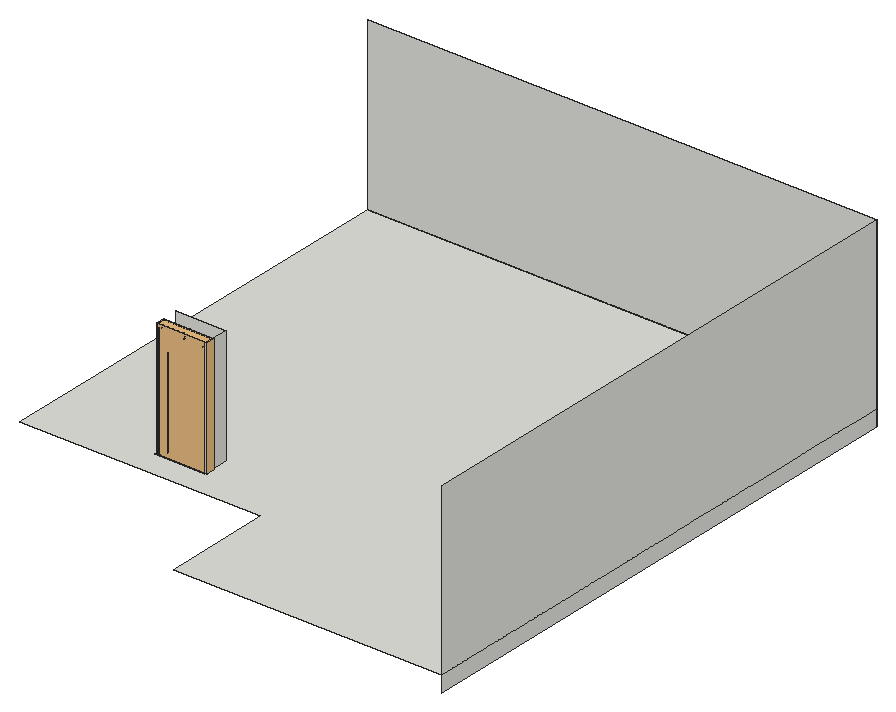
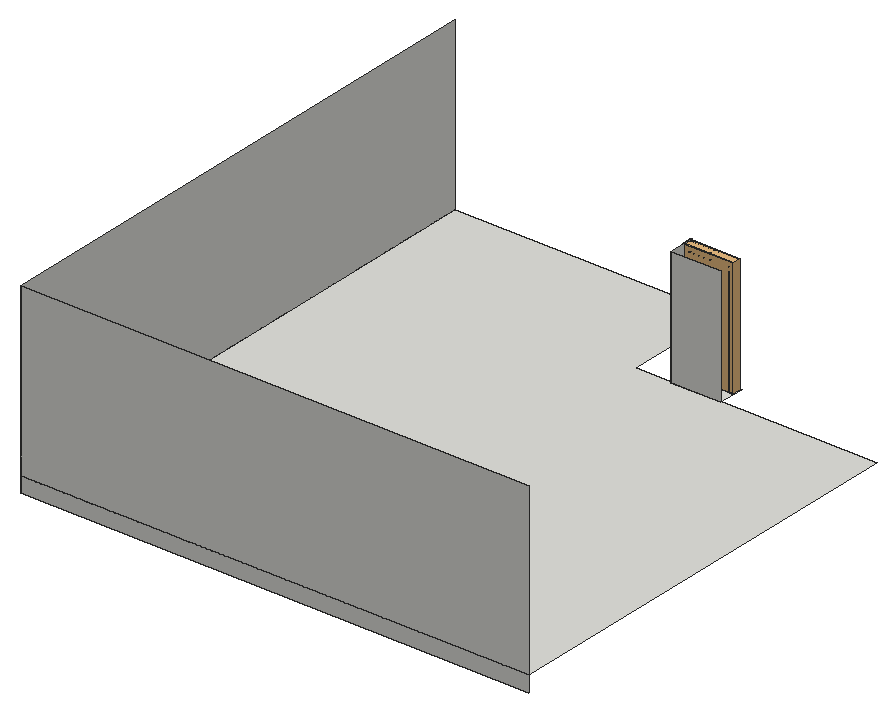
# SketchUp Ruby script. Lengths in inches.
U = 1.inch
M = Sketchup.active_model
def pt(a) = Geom::Point3d.new(a.map { |v| v * U })
def face(e, loops, mat)
  f = e.add_face(loops[0].map { |a| pt(a) })
  loops[1..].each { |l| e.add_face(l.map { |a| pt(a) }).erase! }
  f.material = f.back_material = mat if mat
  f
end
# faces: each face lists its corners as indices into pts; further lists are holes
def faces(e, pts, list, mat = nil) = list.each { |f| face(e, (f[0].is_a?(Array) ? f : [f]).map { |l| l.map { |i| pts[i] } }, mat) }
# xy, xz, yz: faces in a plane at the given z, y or x. An outline is a flat list of corners, or four numbers for a rectangle; further outlines are holes
def ring(l) = l.size == 4 ? [[l[0], l[1]], [l[2], l[1]], [l[2], l[3]], [l[0], l[3]]] : l.each_slice(2).to_a
def flat(e, list, mat, &to3) = list.each { |f| face(e, (f[0].is_a?(Array) ? f : [f]).map { |l| ring(l).map { |u, v| to3.(u, v) } }, mat) }
def xy(e, z, list, mat = nil) = flat(e, list, mat) { |x, y| [x, y, z] }
def xz(e, y, list, mat = nil) = flat(e, list, mat) { |x, z| [x, y, z] }
def yz(e, x, list, mat = nil) = flat(e, list, mat) { |y, z| [x, y, z] }
def lines(e, pts, list) = list.each { |a, b| e.add_line(pt(pts[a]), pt(pts[b])) }
# prism: a flat outline (further loops are holes) pulled along v
def prism(e, loops, v, mat = nil)
  f = face(e, loops, mat); d = Geom::Vector3d.new(v.map { |x| x * U })
  f.pushpull(f.normal.samedirection?(d) ? d.length : -d.length)
end
def box(e, o, s, mat = nil) = prism(e, [[o, [o[0] + s[0], o[1], o[2]], [o[0] + s[0], o[1] + s[1], o[2]], [o[0], o[1] + s[1], o[2]]]], [0, 0, s[2]], mat)
def at(x, y, z, deg = 0) = Geom::Transformation.translation(pt([x, y, z])) * Geom::Transformation.rotation(ORIGIN, Z_AXIS, deg.degrees)
def axes(o, x, y, z) = Geom::Transformation.new([*x, 0, *y, 0, *z, 0, *pt(o).to_a, 1])
def part(name) = M.definitions.add(name)
# library, detail: a bought-in or finely detailed component or shape, given as its bounding box
def library(name, o, s) = part(name).tap { |d| box(d.entities, o, s) }
def detail(e, o, s) = box(e.add_group.entities, o, s)
def put(e, d, t, mat = nil) = e.add_instance(d, t).tap { |i| i.material = mat if mat }
def group(e, t, mat = nil) = e.add_group.tap { |g| g.transformation = t; g.material = mat if mat }.entities
root = M.entities
M.materials.add("Material \#0").color = [86, 53, 35]
M.materials.add("Material \#1").color = [140, 140, 140]
c1 = part("3DGeom~19_Defintion")
xy(c1.entities,0,[[-6.28,-215.79,-994.45,-208.55,-13.52,-208.55],[-994.45,-215.79,-994.45,-208.55,-6.28,-215.79],[-6.28,-215.79,-13.52,-208.55,-13.52,0],[-6.28,-215.79,-13.52,0,-6.28,0],[-13.52,0,-13.52,208.55,-6.28,215.79],
  [-13.52,0,-6.28,215.79,-6.28,0],[-994.45,208.55,-6.28,215.79,-13.52,208.55],[-994.45,208.55,-994.45,215.79,-6.28,215.79]],"Material \#0")
p = [[-13.52,-208.55,0],[-994.45,-208.55,0],[-994.45,-207.81,0.07],[-14.25,-207.81,0.07],[-13.52,-208.55,0],[-14.25,-207.81,0.07],
  [-14.25,0,0.07],[-13.52,0,0],[-13.52,208.55,0],[-14.25,207.81,0.07],[-13.52,208.55,0],[-14.25,207.81,0.07],
  [-994.45,207.81,0.07],[-994.45,208.55,0],[-994.45,-207.21,0.27],[-994.45,-207.21,0.27],[-14.86,-207.21,0.27],[-14.86,-207.21,0.27],
  [-14.86,0,0.27],[-14.86,0,0.27],[-14.86,0,0.27],[-14.86,0,0.27],[-14.86,207.21,0.27],[-14.86,207.21,0.27],
  [-994.45,207.21,0.27],[-994.45,207.21,0.27],[-14.86,-207.21,0.27],[-994.45,-207.21,0.27],[-994.45,-206.74,0.6],[-15.33,-206.74,0.6],
  [-14.86,-207.21,0.27],[-15.33,-206.74,0.6],[-15.33,0,0.6],[-14.86,0,0.27],[-14.86,207.21,0.27],[-15.33,206.74,0.6],
  [-14.86,207.21,0.27],[-15.33,206.74,0.6],[-994.45,206.74,0.6],[-994.45,207.21,0.27],[-994.45,-206.4,1.07],[-15.66,-206.4,1.07],
  [-15.66,-206.4,1.07],[-15.66,0,1.07],[-15.66,206.4,1.07],[-15.66,206.4,1.07],[-994.45,206.4,1.07],[-994.45,-206.2,1.68],
  [-15.86,-206.2,1.68],[-15.86,-206.2,1.68],[-15.86,0,1.68],[-15.86,206.2,1.68],[-15.86,206.2,1.68],[-994.45,206.2,1.68],
  [-994.45,-206.13,2.41],[-15.93,-206.13,2.41],[-15.93,-206.13,2.41],[-15.93,0,2.41],[-15.93,206.13,2.41],[-15.93,206.13,2.41],
  [-994.45,206.13,2.41],[-994.45,-206.13,71.16],[-994.45,-206.22,71.59],[-15.79,-206.28,71.53],[-15.79,-206.28,71.53],[-15.84,0,71.59],
  [-15.93,0,71.16],[-15.79,206.28,71.53],[-15.79,206.28,71.53],[-994.45,206.22,71.59],[-994.45,206.13,71.16],[-15.79,-206.28,71.53],
  [-994.45,-206.48,71.84],[-994.45,-206.9,71.93],[-15.16,-206.9,71.93],[-15.79,-206.28,71.53],[-15.79,-206.28,71.53],[-15.16,-206.9,71.93],
  [-15.16,0,71.93],[-994.45,-206.48,71.84],[-15.59,0,71.84],[-15.79,-206.28,71.53],[-15.59,0,71.84],[-15.79,206.28,71.53],
  [-15.16,206.9,71.93],[-15.59,0,71.84],[-15.79,206.28,71.53],[-994.45,206.48,71.84],[-15.79,206.28,71.53],[-15.16,206.9,71.93],
  [-994.45,206.9,71.93],[-994.45,206.48,71.84],[-15.79,206.28,71.53],[-994.45,-227.27,72.01],[5.41,-227.47,72.33],[4.78,-226.84,71.93],
  [4.78,-226.84,71.93],[5.41,-227.47,72.33],[5.21,0,72.01],[-994.45,-226.84,71.93],[-994.45,-227.27,72.01],[5.21,0,72.01],
  [4.78,0,71.93],[4.78,226.84,71.93],[5.21,0,72.01],[5.21,0,72.01],[5.41,227.47,72.33],[4.78,226.84,71.93],
  [5.41,227.47,72.33],[-994.45,227.27,72.01],[-994.45,227.27,72.01],[-994.45,226.84,71.93],[-994.45,-227.27,72.01],[-994.45,-227.53,72.27],
  [5.41,-227.47,72.33],[5.41,-227.47,72.33],[5.47,0,72.27],[5.21,0,72.01],[5.41,227.47,72.33],[5.41,227.47,72.33],
  [-994.45,227.53,72.27],[-994.45,227.27,72.01],[-994.45,-227.61,72.7],[-994.45,-227.61,74.4375],[-994.45,-227.61,74.4375],[5.55,-227.61,74.4375],
  [5.55,-227.61,74.4375],[5.55,0,74.4375],[5.55,0,72.7],[5.55,227.61,74.4375],[5.55,227.61,74.4375],[-994.45,227.61,74.4375],
  [-994.45,227.61,74.4375],[-994.45,227.61,72.7]]
faces(c1.entities,p,[[0,1,2],[2,3,0],[4,5,6],[6,7,4],[8,7,6],[6,9,8],[10,11,12],[12,13,10],
  [3,2,14],[15,16,3],[5,17,18],[19,6,5],[9,6,20],[21,22,9],[11,23,24],[25,12,11],
  [26,27,28],[28,29,26],[30,31,32],[32,33,30],[34,33,32],[32,35,34],[36,37,38],[38,39,36],
  [29,28,40],[40,41,29],[31,42,43],[43,32,31],[35,32,43],[43,44,35],[37,45,46],[46,38,37],
  [41,40,47],[47,48,41],[42,49,50],[50,43,42],[44,43,50],[50,51,44],[45,52,53],[53,46,45],
  [48,47,54],[54,55,48],[49,56,57],[57,50,49],[51,50,57],[57,58,51],[52,59,60],[60,53,52],
  [61,62,63],[64,65,66],[66,65,67],[68,69,70],[71,72,73],[73,74,75],[76,77,78],[62,79,63],
  [78,80,76],[81,82,65],[83,80,78],[78,84,83],[65,85,86],[68,87,69],[88,89,90],[90,91,92],
  [93,94,95],[96,97,98],[95,99,100],[101,102,96],[103,102,104],[105,106,103],[107,108,109],[110,111,107],
  [112,113,114],[115,116,117],[117,116,118],[119,120,121],[114,122,123],[124,125,114],[113,122,114],[115,126,127],
  [127,128,115],[115,128,116],[118,128,127],[127,129,118],[116,128,118],[119,130,131],[132,133,119],[119,133,120]],"Material \#0")
c2 = part("3DGeom~15_Defintion")
xy(c2.entities,0,[[-961.58,-251.9,-958.5,-248.8125,-961.58,-237.8],[-961.58,-251.9,28.8,-248.8125,-958.5,-248.8125],[-961.58,-251.9,36.25,-251.9,28.8,-248.8125],[36.25,-251.9,19.98,-239.99,28.8,-248.8125],[36.25,-251.9,22.16,-237.8,19.98,-239.99],
  [-958.5,-248.8125,-958.5,-237.8,-961.58,-237.8],[19.98,-239.99,22.16,-237.8,3.36,-223.37],[-958.5,-237.8,-958.5,-223.37,-961.58,-220.28],[-961.58,-237.8,-958.5,-237.8,-961.58,-220.28],[22.16,-237.8,4.64,-220.28,3.36,-223.37],
  [-958.5,-223.37,4.64,-220.28,-961.58,-220.28],[-958.5,-223.37,3.36,-223.37,4.64,-220.28],[5.29,-219.63,8.375,-218.35,5.29,0],[8.375,-218.35,8.375,0,5.29,0],[5.29,0,8.375,0,5.29,219.63],
  [8.375,0,8.375,218.35,5.29,219.63],[8.375,218.35,22.8125,237.15,5.29,219.63],[-961.58,220.28,-958.5,223.37,-961.58,237.8],[-961.58,220.28,3.36,223.37,-958.5,223.37],[-961.58,220.28,4.64,220.28,3.36,223.37],
  [4.64,220.28,19.98,239.99,3.36,223.37],[4.64,220.28,22.16,237.8,19.98,239.99],[-958.5,223.37,-958.5,237.8,-961.58,237.8],[-958.5,237.8,-958.5,248.8125,-961.58,251.9],[-961.58,237.8,-958.5,237.8,-961.58,251.9],
  [22.16,237.8,28.8,248.8125,19.98,239.99],[22.16,237.8,36.25,251.9,28.8,248.8125],[-958.5,248.8125,36.25,251.9,-961.58,251.9],[-958.5,248.8125,28.8,248.8125,36.25,251.9]],"Material \#0")
xy(c2.entities,7.48,[[-962.79,-238.36,23.37,-238.36,-962.79,-219.67],[23.37,-238.36,4.67,-219.67,-962.79,-219.67],[23.37,-238.36,23.37,0,4.67,-219.67],[4.67,-219.67,23.37,0,4.67,0],[23.37,0,23.37,238.36,4.67,219.67],
  [4.67,0,23.37,0,4.67,219.67],[-962.79,219.67,23.37,238.36,-962.79,238.36],[-962.79,219.67,4.67,219.67,23.37,238.36]],"Material \#0")
xy(c2.entities,63.5625,[[-962.79,-238.36,-962.79,-219.67,4.67,-219.67],[-962.79,-238.36,4.67,-219.67,23.37,-238.36],[23.37,-238.36,4.67,-219.67,23.37,0],[4.67,-219.67,4.67,0,23.37,0],[23.37,0,4.67,219.67,23.37,238.36],
  [4.67,0,4.67,219.67,23.37,0],[-962.79,219.67,-962.79,238.36,4.67,219.67],[4.67,219.67,-962.79,238.36,23.37,238.36]],"Material \#0")
xy(c2.entities,69.64,[[-962.79,-219.62,4.63,-219.62,-962.79,-200.32],[4.63,-219.62,-14.68,-200.32,-962.79,-200.32],[4.63,-219.62,4.63,0,-14.68,-200.32],[-14.68,-200.32,4.63,0,-14.68,0],[-14.68,0,4.63,0,-14.68,200.32],
  [4.63,0,4.63,219.62,-14.68,200.32],[-962.79,200.32,-14.68,200.32,4.63,219.62],[-962.79,200.32,4.63,219.62,-962.79,219.62]],"Material \#0")
xy(c2.entities,71.04,[[-961.58,-251.9,-958.5,-248.8125,28.8,-248.8125],[-961.58,-251.9,-961.58,-237.8,-958.5,-248.8125],[-961.58,-251.9,28.8,-248.8125,36.25,-251.9],[36.25,-251.9,19.98,-239.99,22.16,-237.8],[36.25,-251.9,28.8,-248.8125,19.98,-239.99],
  [-958.5,-248.8125,-961.58,-237.8,-958.5,-237.8],[19.98,-239.99,3.36,-223.37,22.16,-237.8],[-958.5,-237.8,-961.58,-220.28,-958.5,-223.37],[-961.58,-237.8,-961.58,-220.28,-958.5,-237.8],[22.16,-237.8,3.36,-223.37,4.64,-220.28],
  [-958.5,-223.37,-961.58,-220.28,4.64,-220.28],[-958.5,-223.37,4.64,-220.28,3.36,-223.37],[5.29,-219.63,5.29,0,8.375,-218.35],[8.375,-218.35,5.29,0,8.375,0],[5.29,0,5.29,219.63,8.375,0],
  [8.375,0,5.29,219.63,8.375,218.35],[8.375,218.35,5.29,219.63,22.8125,237.15],[-961.58,220.28,-958.5,223.37,3.36,223.37],[-961.58,220.28,-961.58,237.8,-958.5,223.37],[-961.58,220.28,3.36,223.37,4.64,220.28],
  [4.64,220.28,3.36,223.37,19.98,239.99],[4.64,220.28,19.98,239.99,22.16,237.8],[-958.5,223.37,-961.58,237.8,-958.5,237.8],[-958.5,237.8,-961.58,251.9,-958.5,248.8125],[-961.58,237.8,-961.58,251.9,-958.5,237.8],
  [22.16,237.8,19.98,239.99,28.8,248.8125],[22.16,237.8,28.8,248.8125,36.25,251.9],[-958.5,248.8125,-961.58,251.9,36.25,251.9],[-958.5,248.8125,36.25,251.9,28.8,248.8125]],"Material \#0")
xz(c2.entities,-238.36,[[-962.79,63.5625,23.37,63.5625,23.37,72.07],[-962.79,63.5625,23.37,72.07,-962.79,72.07]],"Material \#0")
xz(c2.entities,-219.67,[[-962.79,7.48,4.67,7.48,-962.79,63.5625],[4.67,7.48,4.67,63.5625,-962.79,63.5625]],"Material \#0")
xz(c2.entities,219.67,[[-962.79,7.48,-962.79,63.5625,4.67,7.48],[4.67,7.48,-962.79,63.5625,4.67,63.5625]],"Material \#0")
xz(c2.entities,238.36,[[-962.79,63.5625,-962.79,72.07,23.37,72.07],[-962.79,63.5625,23.37,72.07,23.37,63.5625]],"Material \#0")
yz(c2.entities,4.67,[[-219.67,7.48,0,7.48,-219.67,63.5625],[0,7.48,0,63.5625,-219.67,63.5625],[0,7.48,219.67,63.5625,0,63.5625],[0,7.48,219.67,7.48,219.67,63.5625]],"Material \#0")
yz(c2.entities,23.37,[[-238.36,63.5625,0,63.5625,-238.36,72.07],[0,63.5625,0,72.07,-238.36,72.07],[0,63.5625,238.36,63.5625,238.36,72.07],[0,63.5625,238.36,72.07,0,72.07]],"Material \#0")
p = [[36.9,-251.24,0],[37.21,0,-0.16],[34.125,0,-0.14],[36.9,251.24,0],[33.83,243.81,0.02],[33.83,-243.8,0.02],
  [22.8125,-237.15,0],[24.99,-234.97,-0.01],[5.375,-220.37,0],[23.37,-238.36,7.48],[4.67,-219.67,7.48],[4.67,-219.67,7.48],
  [23.37,-238.36,7.48],[23.37,-238.36,0],[4.67,-219.67,7.48],[23.37,-238.36,0],[5.375,-220.37,0],[5.375,-220.37,0],
  [23.37,-238.36,0],[5.29,-219.63,0],[8.375,-218.35,0],[-15.36,-199.64,1.62],[4.67,-219.67,7.48],[5.375,-220.37,0],
  [-13.8,-201.19,0.06],[5.375,-220.37,0],[5.375,-220.37,0],[-14.84,-200.15,0.58],[5.375,-220.37,0],[-13.8,-201.19,0.06],
  [-6.08,-208.92,0],[5.375,-220.37,0],[-13.8,-201.19,0.06],[-6.08,-208.92,0],[-13.8,-201.19,0.06],[5.375,-220.37,0],
  [-6.08,-208.92,0],[-13.8,-201.19,0.06],[-13.09,-201.91,0],[-6.08,-208.92,0],[-13.09,-201.91,0],[-13.8,-201.19,0.06],
  [-15.36,199.64,1.62],[4.67,219.67,7.48],[5.375,220.37,0],[-13.8,201.19,0.06],[5.375,220.37,0],[5.375,220.37,0],
  [4.67,219.67,7.48],[-14.84,200.15,0.58],[5.375,220.37,0],[-13.8,201.19,0.06],[-6.08,208.92,0],[-13.09,201.91,0],
  [-13.8,201.19,0.06],[-6.08,208.92,0],[-13.8,201.19,0.06],[5.375,220.37,0],[-6.08,208.92,0],[5.375,220.37,0],
  [-13.8,201.19,0.06],[-6.08,208.92,0],[-13.8,201.19,0.06],[-13.09,201.91,0],[8.375,218.35,0],[24.99,234.97,-0.01],
  [22.8125,237.15,0],[23.37,238.36,7.48],[23.37,238.36,0],[23.37,238.36,0],[5.375,220.37,0],[5.375,220.37,0],
  [23.37,238.36,7.48],[4.67,219.67,7.48],[5.375,220.37,0],[23.37,238.36,0],[23.37,238.36,7.48],[-13.8,-201.19,0.06],
  [-14.84,-200.15,0.58],[-14.38,-200.61,0.26],[-13.8,-201.19,0.06],[-13.8,-201.19,0.06],[-14.38,-200.61,0.26],[-13.8,201.19,0.06],
  [-14.84,200.15,0.58],[-13.8,201.19,0.06],[-14.38,200.61,0.26],[-14.38,200.61,0.26],[-13.8,201.19,0.06],[4.63,-219.62,69.64],
  [4.63,-219.62,69.64],[-15.42,-199.57,9.43],[-15.36,-199.64,1.62],[-15.16,-199.83,1.04],[-15.16,-199.83,1.04],[-15.16,199.83,1.04],
  [-15.36,199.64,1.62],[-15.16,199.83,1.04],[-15.42,199.57,9.43],[4.63,219.62,69.64],[4.67,219.67,7.48],[4.63,219.62,69.64],
  [4.63,-219.62,69.64],[4.67,-219.67,63.5625],[4.67,-219.67,63.5625],[4.67,-219.67,7.48],[-15.28,-199.71,69.25],[4.63,-219.62,69.64],
  [-15.42,-199.57,9.43],[-15.28,-199.71,69.25],[-15.42,-199.57,2.34],[-15.42,-199.57,2.34],[-15.42,199.57,2.34],[-15.42,199.57,9.43],
  [-15.28,199.71,69.25],[-15.28,199.71,69.25],[4.63,219.62,69.64],[4.63,219.62,69.64],[4.67,219.67,63.5625],[4.67,219.67,63.5625],
  [-15.42,199.57,2.34],[4.67,-219.67,63.5625],[4.63,-219.62,69.64],[4.67,219.67,7.48],[4.67,219.67,63.5625],[4.63,219.62,69.64],
  [4.63,-219.62,69.64],[-15.28,-199.71,69.25],[-15.28,-199.71,69.25],[-15.42,-199.57,48.99],[-15.42,-199.57,48.99],[-15.28,-199.71,69.25],
  [-15.42,199.57,48.99],[-15.28,199.71,69.25],[-15.28,199.71,69.25],[-15.42,199.57,48.99],[4.63,219.62,69.64],[4.63,-219.62,69.64],
  [23.37,-238.36,72.07],[4.67,-219.67,63.5625],[4.67,-219.67,63.5625],[23.37,-238.36,63.5625],[23.37,-238.36,72.07],[4.67,-219.67,63.5625],
  [5.24,-220.23,70.03],[23.37,-238.36,72.07],[23.37,-238.36,63.5625],[4.67,-219.67,63.5625],[4.67,-219.67,63.5625],[4.63,-219.62,69.64],
  [4.63,219.62,69.64],[23.37,238.36,72.07],[4.67,219.67,63.5625],[4.67,219.67,63.5625],[5.24,220.23,70.03],[4.63,219.62,69.64],
  [23.37,238.36,63.5625],[4.67,219.67,63.5625],[4.67,219.67,63.5625],[23.37,238.36,63.5625],[23.37,238.36,72.07],[4.67,219.67,63.5625],
  [23.37,238.36,72.07],[4.63,-219.62,69.64],[-14.68,-200.32,69.64],[-15.28,-199.71,69.25],[-15.28,-199.71,69.25],[-14.68,-200.32,69.64],
  [4.63,-219.62,69.64],[-15.28,199.71,69.25],[-14.68,200.32,69.64],[4.63,219.62,69.64],[4.63,219.62,69.64],[-14.68,200.32,69.64],
  [4.63,-219.62,69.64],[5.24,-220.23,70.03],[23.37,-238.36,72.07],[4.63,219.62,69.64],[5.24,220.23,70.03],[5.375,-220.37,72.07],
  [5.375,-220.37,72.07],[23.37,-238.36,72.07],[5.375,220.37,72.07],[23.37,238.36,72.07],[5.375,220.37,72.07],[33.83,-243.8,71.03],
  [36.9,-251.24,71.04],[22.8125,-237.15,71.04],[34.125,0,71.19],[37.21,0,71.2],[24.99,-234.97,71.05],[5.29,-219.63,71.04],
  [8.375,-218.35,71.04],[33.83,243.81,71.03],[36.9,251.24,71.04],[22.8125,237.15,71.04],[24.99,234.97,71.05],[8.375,218.35,71.04]]
faces(c2.entities,p,[[0,1,2],[1,3,4],[4,2,1],[2,5,0],[6,0,5],[5,7,6],[8,9,10],[11,12,13],
  [14,15,16],[17,18,9],[19,6,7],[7,20,19],[21,22,23],[24,21,25],[26,10,27],[28,27,29],
  [30,31,32],[33,34,35],[36,37,38],[39,40,41],[42,43,44],[45,42,46],[47,48,49],[50,49,51],
  [52,53,54],[55,56,57],[58,59,60],[61,62,63],[64,65,66],[43,67,68],[43,69,70],[71,72,73],
  [74,75,76],[3,66,65],[65,4,3],[77,78,21],[27,79,80],[81,82,78],[83,84,42],[85,86,84],
  [49,87,88],[10,89,27],[90,91,27],[92,93,27],[91,92,27],[78,94,21],[84,95,42],[96,97,49],
  [98,96,49],[99,98,49],[100,101,49],[21,102,103],[21,104,105],[21,106,107],[21,108,109],[91,110,92],
  [21,111,108],[42,112,113],[42,113,114],[42,115,116],[42,117,118],[42,119,43],[98,120,96],[10,121,122],
  [123,124,125],[126,127,91],[128,129,91],[108,130,131],[113,132,133],[134,135,98],[136,134,98],[137,138,139],
  [140,141,142],[143,142,144],[145,146,147],[148,144,149],[150,151,152],[153,154,155],[151,156,157],[158,159,160],
  [161,162,154],[163,164,165],[166,167,168],[169,170,171],[172,173,134],[174,175,176],[177,178,151],[142,179,144],
  [175,180,181],[178,182,151],[183,184,154],[185,186,187],[186,185,188],[188,189,186],[187,190,185],[190,187,191],
  [191,192,190],[189,188,193],[193,194,189],[195,196,197],[196,195,194],[194,193,196]],"Material \#0")
c3 = part("3DGeom~22_Defintion")
xz(c3.entities,-210.625,[[-1016.13,2.47,-1016.13,9.96,-16.28,2.47],[-16.28,2.47,-1016.13,9.96,-16.28,9.96],[-1016.13,9.96,-1016.13,51.7,-16.28,51.7],[-1016.13,9.96,-16.28,51.7,-16.28,9.96],[-1016.13,51.7,-1016.13,72.71,-16.28,51.7]],"Material \#0")
xz(c3.entities,210.625,[[-1016.13,2.47,-16.28,2.47,-1016.13,9.96],[-16.28,2.47,-16.28,9.96,-1016.13,9.96],[-1016.13,9.96,-16.28,51.7,-1016.13,51.7],[-1016.13,9.96,-16.28,9.96,-16.28,51.7],[-1016.13,51.7,-16.28,51.7,-1016.13,72.71]],"Material \#0")
yz(c3.entities,-16.28,[[-210.625,2.47,-210.625,9.96,0,9.96],[-210.625,2.47,0,9.96,0,2.47],[0,2.47,0,9.96,210.625,2.47],[210.625,2.47,0,9.96,210.625,9.96],[-210.625,9.96,-210.625,51.7,0,51.7],
  [-210.625,9.96,0,51.7,0,9.96],[0,9.96,0,51.7,210.625,9.96],[210.625,9.96,0,51.7,210.625,51.7],[-210.625,51.7,0,72.71,0,51.7],[0,51.7,0,72.71,210.625,51.7]],"Material \#0")
p = [[-1016.13,-210.625,72.71],[-16.13,-210.77,73.09],[-16.28,-210.625,51.7],[-16.28,-210.625,51.7],[-16.13,-210.77,73.09],[-16.28,0,72.71],
  [-16.13,210.77,73.09],[-16.28,210.625,51.7],[-16.28,210.625,51.7],[-16.13,210.77,73.09],[-1016.13,210.625,72.71]]
faces(c3.entities,p,[[0,1,2],[3,4,5],[5,6,7],[8,9,10]],"Material \#0")
c4 = library("3DGeom~16_Defintion",[-962.62,-252.34,-11.22],[1000,504.68,93.46])
c5 = part("3DGeom~17_Defintion")
yz(c5.entities,-1908.8,[[-436.03,-21.87,-436.73,-21.5,-435.91,-21.83],[436.03,-21.87,435.91,-21.83,436.73,-21.5],[-435.91,-21.83,-436.73,-21.5,-436.15,-21.125],[-435.91,-21.83,-436.15,-21.125,-435.87,-21.72],[435.91,-21.83,435.87,-21.72,436.15,-21.125],
  [435.91,-21.83,436.15,-21.125,436.73,-21.5],[-436.73,-21.5,-484.73,-21.37,-436.15,-1.11],[-471.46,-21.5,-484.73,-21.37,-436.73,-21.5],[-477.2,-21.5,-484.73,-21.37,-471.46,-21.5],[-481.82,-21.5,-484.73,-21.37,-477.2,-21.5],
  [-436.73,-21.5,-436.15,-1.11,-436.15,-21.125],[436.73,-21.5,436.15,-21.125,471.46,-21.5],[471.46,-21.5,436.15,-21.125,477.2,-21.5],[477.2,-21.5,436.15,-21.125,499.98,-0.85],[477.2,-21.5,499.98,-0.85,481.82,-21.5],
  [481.82,-21.5,487.35,-21,484.73,-21.37],[481.82,-21.5,491.8,-19.52,487.35,-21],[481.82,-21.5,497.64,-13.67,491.8,-19.52],[481.82,-21.5,499.98,-0.85,497.64,-13.67],[-484.73,-21.37,-498.5,-11.58,-499.84,-0.37],
  [-484.73,-21.37,-499.84,-0.37,-499.4,-0.5],[-484.73,-21.37,-499.4,-0.5,-436.15,-1.11],[-484.73,-21.37,-493.63,-18.42,-498.5,-11.58],[-484.73,-21.37,-489.71,-20.375,-493.63,-18.42],[-484.73,-21.37,-487.35,-21,-489.71,-20.375],
  [436.15,-21.125,436.15,-1.11,436.73,-0.74],[436.15,-21.125,436.73,-0.74,499.98,-0.85],[487.35,-21,491.8,-19.52,489.71,-20.375],[-489.71,-20.375,-491.8,-19.52,-493.63,-18.42],[491.8,-19.52,495.21,-17.08,493.63,-18.42],
  [491.8,-19.52,497.64,-13.67,495.21,-17.08],[-493.63,-18.42,-496.54,-15.5,-498.5,-11.58],[-493.63,-18.42,-495.21,-17.08,-496.54,-15.5],[495.21,-17.08,497.64,-13.67,496.54,-15.5],[-496.54,-15.5,-497.64,-13.67,-498.5,-11.58],
  [497.64,-13.67,499.125,-9.22,498.5,-11.58],[497.64,-13.67,499.625,-3.69,499.125,-9.22],[497.64,-13.67,499.98,-0.85,499.625,-3.69],[-498.5,-11.58,-499.625,-3.69,-499.84,-0.37],[-498.5,-11.58,-499.5,-6.6,-499.625,-3.69],
  [-498.5,-11.58,-499.125,-9.22,-499.5,-6.6],[499.125,-9.22,499.625,-3.69,499.5,-6.6],[-499.625,-3.69,-499.98,-0.85,-500,-0.52],[-499.625,-3.69,-500,-0.52,-499.84,-0.37],[-436.15,-1.11,-499.4,-0.5,-471.46,-0.74],
  [-436.15,-1.11,-471.46,-0.74,-436.73,-0.74],[-436.15,-1.11,-436.73,-0.74,-435.91,-0.41],[-436.15,-1.11,-435.91,-0.41,-435.87,-0.52],[436.15,-1.11,435.87,-0.52,435.91,-0.41],[436.15,-1.11,435.91,-0.41,436.73,-0.74],
  [499.98,-0.85,436.73,-0.74,471.46,-0.74],[499.98,-0.85,471.46,-0.74,499.4,-0.5],[499.98,-0.85,499.4,-0.5,499.96,-0.41],[499.98,-0.85,499.96,-0.41,500,-0.52],[-436.73,-0.74,-436.03,-0.37,-435.91,-0.41],
  [436.73,-0.74,435.91,-0.41,436.03,-0.37],[-500,-0.52,-499.96,-0.41,-499.84,-0.37],[499.4,-0.5,499.84,-0.37,499.96,-0.41],[-499.84,141.21,-499.96,141.25,-499.4,141.35],[-436.03,141.21,-436.73,141.59,-435.91,141.25],
  [436.03,141.21,435.91,141.25,436.73,141.59],[499.84,141.21,484.73,162.21,498.5,152.42],[499.84,141.21,499.4,141.35,484.73,162.21],[499.84,141.21,498.5,152.42,499.625,144.53],[499.84,141.21,499.625,144.53,500,141.37],
  [499.84,141.21,500,141.37,499.96,141.25],[-499.96,141.25,-500,141.37,-499.98,141.69],[-499.96,141.25,-499.98,141.69,-499.4,141.35],[-435.91,141.25,-436.73,141.59,-436.15,141.96],[-435.91,141.25,-436.15,141.96,-435.87,141.37],
  [435.91,141.25,435.87,141.37,436.15,141.96],[435.91,141.25,436.15,141.96,436.73,141.59],[-499.4,141.35,-499.98,141.69,-471.46,141.59],[499.4,141.35,436.15,141.96,484.73,162.21],[499.4,141.35,471.46,141.59,436.15,141.96],
  [500,141.37,499.625,144.53,499.98,141.69],[-436.73,141.59,-499.98,141.69,-436.15,161.97],[-471.46,141.59,-499.98,141.69,-436.73,141.59],[-436.73,141.59,-436.15,161.97,-436.15,141.96],[436.73,141.59,436.15,141.96,471.46,141.59],
  [-499.98,141.69,-477.2,162.34,-436.15,161.97],[-499.98,141.69,-481.82,162.34,-477.2,162.34],[-499.98,141.69,-497.64,154.51,-481.82,162.34],[-499.98,141.69,-499.625,144.53,-497.64,154.51],[436.15,141.96,436.15,161.97,436.73,162.34],
  [436.15,141.96,436.73,162.34,484.73,162.21],[-499.625,144.53,-499.125,150.07,-497.64,154.51],[-499.625,144.53,-499.5,147.44,-499.125,150.07],[499.625,144.53,498.5,152.42,499.5,147.44],[499.5,147.44,498.5,152.42,499.125,150.07],
  [-499.125,150.07,-498.5,152.42,-497.64,154.51],[498.5,152.42,484.73,162.21,493.63,159.26],[498.5,152.42,493.63,159.26,496.54,156.34],[498.5,152.42,496.54,156.34,497.64,154.51],[-497.64,154.51,-491.8,160.36,-481.82,162.34],
  [-497.64,154.51,-495.21,157.92,-491.8,160.36],[-497.64,154.51,-496.54,156.34,-495.21,157.92],[496.54,156.34,493.63,159.26,495.21,157.92],[-495.21,157.92,-493.63,159.26,-491.8,160.36],[493.63,159.26,484.73,162.21,489.71,161.22],
  [493.63,159.26,489.71,161.22,491.8,160.36],[-491.8,160.36,-487.35,161.84,-481.82,162.34],[-491.8,160.36,-489.71,161.22,-487.35,161.84],[489.71,161.22,484.73,162.21,487.35,161.84],[-487.35,161.84,-484.73,162.21,-481.82,162.34],
  [-436.15,161.97,-477.2,162.34,-471.46,162.34],[-436.15,161.97,-471.46,162.34,-436.73,162.34],[-436.15,161.97,-436.73,162.34,-435.91,162.68],[-436.15,161.97,-435.91,162.68,-435.87,162.56],[436.15,161.97,435.87,162.56,435.91,162.68],
  [436.15,161.97,435.91,162.68,436.73,162.34],[484.73,162.21,436.73,162.34,471.46,162.34],[484.73,162.21,471.46,162.34,477.2,162.34],[484.73,162.21,477.2,162.34,481.82,162.34],[-436.73,162.34,-436.03,162.72,-435.91,162.68],
  [436.73,162.34,435.91,162.68,436.03,162.72]],"Material \#0")
c6 = part("3DGeom~18_Defintion")
xz(c6.entities,-241.71,[[-976.3,0,23.7,0,23.7,7.58],[-976.3,0,23.7,7.58,-976.3,7.58]],"Material \#0")
xz(c6.entities,241.71,[[-976.3,0,-976.3,7.58,23.7,7.58],[-976.3,0,23.7,7.58,23.7,0]],"Material \#0")
yz(c6.entities,23.7,[[-241.71,0,0,0,-241.71,7.58],[0,0,0,7.58,-241.71,7.58],[0,0,241.71,0,241.71,7.58],[0,0,241.71,7.58,0,7.58]],"Material \#0")
c7 = part("3DGeom~20_Defintion")
xy(c7.entities,0,[[-976.3,-241.71,-976.3,-223.46,23.7,-241.71],[23.7,-241.71,-976.3,-223.46,5.45,-223.46],[23.7,-241.71,5.45,-223.46,5.45,0],[23.7,-241.71,5.45,0,23.7,0],[-976.3,-223.46,-976.3,-211.85,5.45,-223.46],
  [5.45,-223.46,-976.3,-211.85,-6.16,-211.85],[5.45,-223.46,-6.16,-211.85,-6.16,0],[5.45,-223.46,-6.16,0,5.45,0],[-6.16,0,-6.16,211.85,5.45,223.46],[-6.16,0,5.45,223.46,5.45,0],
  [5.45,0,23.7,241.71,23.7,0],[5.45,0,5.45,223.46,23.7,241.71],[-976.3,211.85,-976.3,223.46,5.45,223.46],[-976.3,211.85,5.45,223.46,-6.16,211.85],[-976.3,223.46,-976.3,241.71,23.7,241.71],
  [-976.3,223.46,23.7,241.71,5.45,223.46]],"Material \#0")
xy(root,0,[[169.98,37.59,360,37.59,360,421.59,0,421.59,0,114.72,169.98,114.72]])
xy(root,12.9,[[95,114.72,130.44,133.09]])
xz(root,117.63,[[101.39,47.08,101.49,47.1,101.39,47.09],[101.39,47.08,101.5,47.09,101.49,47.1],[101.5,47.09,101.59,47.13,101.49,47.1],[101.59,47.12,101.68,47.17,101.68,47.18],[101.68,47.17,101.76,47.24,101.68,47.18],
  [101.43,47.26,101.46,47.27,101.46,47.28],[101.43,47.26,101.46,47.28,101.43,47.27],[101.46,47.27,101.48,47.3,101.46,47.28],[101.46,47.27,101.49,47.29,101.48,47.3],[101.49,47.29,101.51,47.32,101.48,47.3],
  [101.49,47.29,101.52,47.31,101.51,47.32],[101.52,47.31,101.53,47.34,101.51,47.32],[101.52,47.31,101.54,47.34,101.53,47.34],[101.53,47.34,101.54,47.34,101.55,47.375],[101.54,47.34,101.56,47.37,101.55,47.375],
  [101.55,47.59,101.56,47.6,101.53,47.62],[101.56,47.6,101.54,47.625,101.53,47.62],[101.53,47.62,101.54,47.625,101.51,47.64],[101.54,47.625,101.52,47.65,101.51,47.64],[101.51,47.64,101.52,47.65,101.48,47.67],
  [101.52,47.65,101.49,47.68,101.48,47.67],[101.48,47.67,101.49,47.68,101.46,47.68],[101.46,47.68,101.46,47.69,101.43,47.69],[101.46,47.68,101.49,47.68,101.46,47.69],[101.43,47.69,101.46,47.69,101.43,47.7]],"Material \#1")
xz(root,133.09,[[95,12.9,130.44,95.77]])
xz(root,421.59,[[0,-11.1875,360,0],[0,0,360,120]])
yz(root,130.44,[[114.72,12.9,133.09,95.77]])
yz(root,360,[[37.59,-11.1875,421.59,0],[37.59,0,421.59,120]])
put(root,c1,axes([113.53,121.22,92.68],[0,0,0.08022],[0.06797,0,0],[0,-0.06357,0]),"Material \#0")
put(root,c2,axes([113.53,121.22,92.68],[0,0,0.08286],[0.07021,0,0],[0,-0.06566,0]),"Material \#0")
put(root,c3,axes([113.53,121.22,92.68],[0,0,0.07851],[0.06652,0,0],[0,-0.06222,0]),"Material \#0")
put(root,c4,axes([113.53,121.22,92.68],[0,0,0.08287],[0.07022,0,0],[0,-0.06568,0]),"Material \#0")
put(root,c5,axes([113.53,121.22,92.68],[0,0,0.04179],[0.03541,0,0],[0,-0.03312,0]),"Material \#0")
put(root,c6,axes([113.53,121.22,92.68],[0,0,0.08171],[0.06923,0,0],[0,-0.06476,0]),"Material \#0")
put(root,c7,axes([113.53,121.22,92.68],[0,0,0.08171],[0.06923,0,0],[0,-0.06476,0]),"Material \#0")
